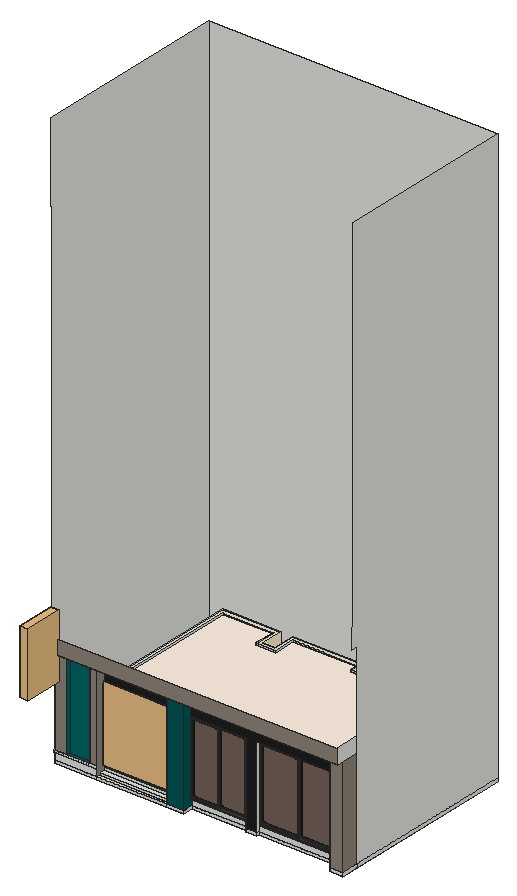
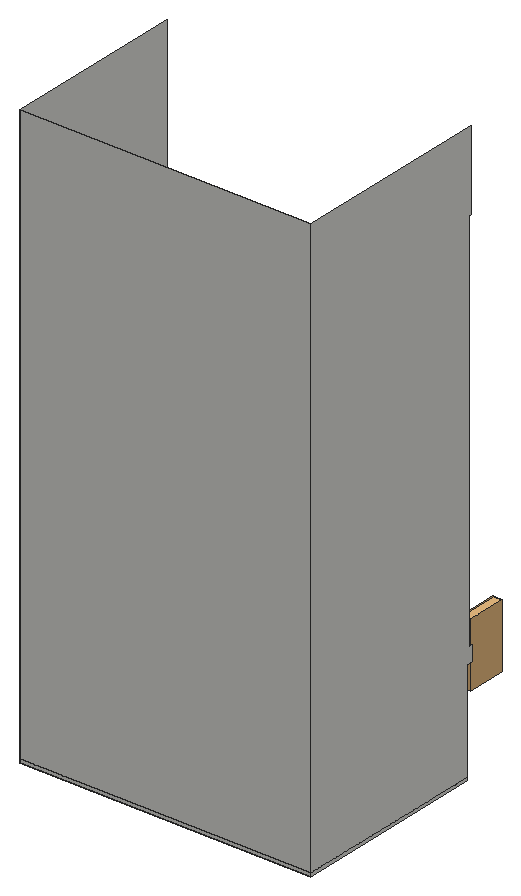
# SketchUp Ruby script. Lengths in inches.
U = 1.inch
M = Sketchup.active_model
def pt(a) = Geom::Point3d.new(a.map { |v| v * U })
def face(e, loops, mat)
  f = e.add_face(loops[0].map { |a| pt(a) })
  loops[1..].each { |l| e.add_face(l.map { |a| pt(a) }).erase! }
  f.material = f.back_material = mat if mat
  f
end
# faces: each face lists its corners as indices into pts; further lists are holes
def faces(e, pts, list, mat = nil) = list.each { |f| face(e, (f[0].is_a?(Array) ? f : [f]).map { |l| l.map { |i| pts[i] } }, mat) }
# xy, xz, yz: faces in a plane at the given z, y or x. An outline is a flat list of corners, or four numbers for a rectangle; further outlines are holes
def ring(l) = l.size == 4 ? [[l[0], l[1]], [l[2], l[1]], [l[2], l[3]], [l[0], l[3]]] : l.each_slice(2).to_a
def flat(e, list, mat, &to3) = list.each { |f| face(e, (f[0].is_a?(Array) ? f : [f]).map { |l| ring(l).map { |u, v| to3.(u, v) } }, mat) }
def xy(e, z, list, mat = nil) = flat(e, list, mat) { |x, y| [x, y, z] }
def xz(e, y, list, mat = nil) = flat(e, list, mat) { |x, z| [x, y, z] }
def yz(e, x, list, mat = nil) = flat(e, list, mat) { |y, z| [x, y, z] }
def lines(e, pts, list) = list.each { |a, b| e.add_line(pt(pts[a]), pt(pts[b])) }
# prism: a flat outline (further loops are holes) pulled along v
def prism(e, loops, v, mat = nil)
  f = face(e, loops, mat); d = Geom::Vector3d.new(v.map { |x| x * U })
  f.pushpull(f.normal.samedirection?(d) ? d.length : -d.length)
end
def box(e, o, s, mat = nil) = prism(e, [[o, [o[0] + s[0], o[1], o[2]], [o[0] + s[0], o[1] + s[1], o[2]], [o[0], o[1] + s[1], o[2]]]], [0, 0, s[2]], mat)
def at(x, y, z, deg = 0) = Geom::Transformation.translation(pt([x, y, z])) * Geom::Transformation.rotation(ORIGIN, Z_AXIS, deg.degrees)
def axes(o, x, y, z) = Geom::Transformation.new([*x, 0, *y, 0, *z, 0, *pt(o).to_a, 1])
def part(name) = M.definitions.add(name)
# library, detail: a bought-in or finely detailed component or shape, given as its bounding box
def library(name, o, s) = part(name).tap { |d| box(d.entities, o, s) }
def detail(e, o, s) = box(e.add_group.entities, o, s)
def put(e, d, t, mat = nil) = e.add_instance(d, t).tap { |i| i.material = mat if mat }
def group(e, t, mat = nil) = e.add_group.tap { |g| g.transformation = t; g.material = mat if mat }.entities
root = M.entities
M.materials.add("Brown Tiles 240cm").color = [174, 145, 135]
M.materials.add("Glass_Tinted_Gray").color = [0, 0, 0]
M.materials["Glass_Tinted_Gray"].alpha = 0.125
M.materials.add("Heather_Band").color = [142, 133, 122]
M.materials.add("[0135_DarkGray]").color = [81, 81, 81]
M.materials.add("[Color C02]").color = [255, 240, 226]
M.materials.add("[Color D01]").color = [255, 242, 204]
M.materials.add("[Color H08]").color = [0, 84, 84]
M.materials.add("[Color H08]1").color = [0, 102, 102]
M.materials.add("[Color M01]1").color = [226, 226, 226]
M.materials.add("[Color M08]").color = [30, 30, 30]
M.materials.add("[Mirror 02]").color = [229, 229, 229]
M.materials.add("[Terrazzo Light Blue]").color = [196, 214, 227]
c1 = part("PENTEK_RP Fineline 50S_Sliding_DoorCase_E1")
box(c1.entities,[0,0,0],[1.51,3.66,99.27],"[0135_DarkGray]")
c2 = part("PENTEK_RP Fineline 50S_SlidingDooe_Case_E2")
box(c2.entities,[0,0,0],[96.25,3.66,1.51],"[0135_DarkGray]")
c3 = part("pentek_RP Fineline 50S_SlidingDoor_Case")
put(c3.entities,c1,at(97.76,0,0))
put(c3.entities,c2,at(1.51,0,0))
put(c3.entities,c1,at(0,0,0))
put(c3.entities,c2,at(1.51,0,97.76))
c4 = part("PENTEK_RP Fineline 50S_SlidingDoor_GlazingBead_2")
box(c4.entities,[0,0,0],[0.56,0.59,94.39],"[0135_DarkGray]")
c5 = part("PENTEK_RP Fineline 50S_SlidingDoor_Glass")
box(c5.entities,[0,0,0],[46.58,0.16,94.39],"Glass_Tinted_Gray")
c6 = part("PENTEK_RP Fineline 50S_SlidingDoor_GlazingBead")
box(c6.entities,[0,0,0],[45.47,0.59,0.56],"[0135_DarkGray]")
c7 = part("PENTEK_RP Fineline 50S_SlidingDoor_Leaf_E1")
xy(c7.entities,0,[[0,0,0.93,1.97],[0.93,1.57,1.49,1.97]],"[0135_DarkGray]")
xy(c7.entities,96.25,[[0,0,0.93,0,0.93,1.57,1.49,1.57,1.49,1.97,0,1.97]],"[0135_DarkGray]")
xz(c7.entities,0,[[0,0,0.93,96.25]],"[0135_DarkGray]")
xz(c7.entities,1.57,[[0.93,0,1.49,95.32],[0.93,95.32,1.49,96.25]],"[0135_DarkGray]")
xz(c7.entities,1.97,[[0,0,1.49,96.25]],"[0135_DarkGray]")
yz(c7.entities,0,[[0,0,1.97,96.25]],"[0135_DarkGray]")
yz(c7.entities,0.93,[[0,0,1.57,0.93],[0,0.93,1.57,95.32],[0,95.32,1.57,96.25]],"[0135_DarkGray]")
yz(c7.entities,1.49,[[1.57,0,1.97,95.32],[1.57,95.32,1.97,96.25]],"[0135_DarkGray]")
c8 = part("PENTEK_RP Fineline 50S_SlidingDoor_Leaf_E2")
xy(c8.entities,0,[[0,0,0,1.57,0.56,1.57,0.56,1.97,46.02,1.97,46.02,1.57,46.58,1.57,46.58,0]],"[0135_DarkGray]")
xy(c8.entities,0.93,[[0,0,46.58,1.57]],"[0135_DarkGray]")
xy(c8.entities,1.49,[[0.56,1.57,46.02,1.97]],"[0135_DarkGray]")
xz(c8.entities,0,[[0,0,46.58,0.93]],"[0135_DarkGray]")
xz(c8.entities,1.57,[[0,0,0.56,0.93],[46.02,0,46.58,0.93],[0.56,0.93,46.02,1.49]],"[0135_DarkGray]")
xz(c8.entities,1.97,[[0.56,0,46.02,1.49]],"[0135_DarkGray]")
yz(c8.entities,0,[[0,0,1.57,0.93]],"[0135_DarkGray]")
yz(c8.entities,0.56,[[1.57,0,1.97,0.93],[1.57,0.93,1.97,1.49]],"[0135_DarkGray]")
yz(c8.entities,46.02,[[1.57,0,1.97,0.93],[1.57,0.93,1.97,1.49]],"[0135_DarkGray]")
yz(c8.entities,46.58,[[0,0,1.57,0.93]],"[0135_DarkGray]")
c9 = part("PENTEK_RP Fineline S_SlidingDoor_Leaf1")
put(c9.entities,c4,at(0.93,0,0.93))
put(c9.entities,c4,at(46.96,0,0.93))
put(c9.entities,c5,at(1.49,1.42,0.93))
put(c9.entities,c6,at(1.49,0,0.93))
put(c9.entities,c5,at(1.49,0.59,0.93),"[Terrazzo Light Blue]")
put(c9.entities,c7,at(0,0,0))
put(c9.entities,c7,axes([48.44,0,0],[-1,0,0],[0,1,0],[0,0,1]))
put(c9.entities,c8,axes([0.93,0,96.25],[1,0,0],[0,1,0],[0,0,-1]))
put(c9.entities,c8,at(0.93,0,0))
put(c9.entities,c6,at(1.49,0,94.77))
c10 = part("PENTEK_RP Fineline 50S_SlidingDoor_Leaf2")
put(c10.entities,c5,at(1.49,1.42,0.93))
put(c10.entities,c6,at(1.49,0,94.77))
put(c10.entities,c4,at(46.96,0,0.93))
put(c10.entities,c5,at(1.49,0.59,0.93),"[Mirror 02]")
put(c10.entities,c4,at(0.93,0,0.93))
put(c10.entities,c7,at(0,0,0))
put(c10.entities,c7,axes([48.44,0,0],[-1,0,0],[0,1,0],[0,0,1]))
put(c10.entities,c6,at(1.49,0,0.93))
put(c10.entities,c8,axes([0.93,0,96.25],[1,0,0],[0,1,0],[0,0,-1]))
put(c10.entities,c8,at(0.93,0,0))
c11 = part("PENTEK - Slimmest Steel Sliding Door / Window\#1")
put(c11.entities,c3,at(0,-1.88,-0.09))
put(c11.entities,c9,at(1.51,-2.27,1.42))
put(c11.entities,c10,at(49.32,-0.3,1.42))
c12 = library("Glass+Door",[0,0,0],[72,3.54,96])
c13 = library("Building Sign 162 041",[-35.6,-7.14,-59.53],[35.45,14.28,119.05])
xy(root,0,[[0,13.61,0,372.45,534.76,372.45,534.76,13.61,510.42,13.61,510.42,32.73,363.26,32.73,363.26,29.02,342.26,29.02,342.26,32.73,239.23,32.73,239.23,13.61]])
xy(root,5.66,[[0,13.61,79,13.61,79,19.17,208.34,19.17,208.34,13.61,239.23,13.61,239.23,32.73,342.26,32.73,342.26,29.02,363.26,29.02,363.26,32.73,510.42,32.73,510.42,13.61,534.76,13.61,534.76,372.45,0,372.45],[79,13.61,208.34,19.17]])
xy(root,9.57,[[79,19.17,208.34,29.02]])
xy(root,14.73,[[79,29.02,208.34,31.95],[239.23,32.73,342.26,34.58],[363.26,32.73,510.42,34.58]])
xy(root,17.05,[[79,29.02,208.34,31.95],[239.23,32.73,342.26,34.58],[363.26,32.73,510.42,34.58]])
xy(root,19.11,[[0,12.67,79,13.61]])
xy(root,19.11,[[79,29.02,208.34,29.02,208.34,37.55,239.23,37.55,239.23,32.73,342.26,32.73,342.26,37.55,363.26,37.55,363.26,32.73,510.42,32.73,510.42,74.25,497.11,74.25,497.11,304.42,361.29,304.42,361.29,287.67,342.26,287.67,342.26,304.42,208.34,304.42,208.34,263.36,186.47,263.36,186.47,304.42,79,304.42]],"Brown Tiles 240cm")
xy(root,23,[[0,12.67,23.3125,13.61],[65.03,12.67,79,13.61]])
xy(root,23,[[23.3125,12.67,65.03,19.67]],"[Color H08]1")
xy(root,152.6,[[85.77,35.79,85.77,297.65,179.69,297.65,179.69,256.58,215.12,256.58,215.12,297.65,335.48,297.65,335.48,280.9,368.07,280.9,368.07,297.65,490.33,297.65,490.33,67.47,503.64,67.47,503.64,35.79,370.03,35.79,370.03,44.32,335.48,44.32,335.48,35.79,246,35.79,246,44.32,201.57,44.32,201.57,35.79]],"[Color C02]")
xy(root,155.66,[[[79,29.02,79,304.42,186.47,304.42,186.47,263.36,208.34,263.36,208.34,304.42,342.26,304.42,342.26,287.67,361.29,287.67,361.29,304.42,497.11,304.42,497.11,74.25,510.42,74.25,510.42,29.02,363.26,29.02,363.26,37.55,342.26,37.55,342.26,29.02,239.23,29.02,239.23,37.55,208.34,37.55,208.34,29.02],[85.77,35.79,201.57,35.79,201.57,44.32,246,44.32,246,35.79,335.48,35.79,335.48,44.32,370.03,44.32,370.03,35.79,503.64,35.79,503.64,67.47,490.33,67.47,490.33,297.65,368.07,297.65,368.07,280.9,335.48,280.9,335.48,297.65,215.12,297.65,215.12,256.58,179.69,256.58,179.69,297.65,85.77,297.65]]])
xy(root,187.02,[[23.3125,13.61,65.03,19.67]],"[Color H08]1")
xy(root,190.91,[[0,1.33,0,13.61,79,13.61,79,29.02,208.34,29.02,208.34,13.61,239.23,13.61,239.23,29.02,510.42,29.02,510.42,13.61,534.76,13.61,534.76,1.33]],"Heather_Band")
xz(root,1.33,[[0,190.91,534.76,216.59]],"Heather_Band")
xz(root,12.67,[[0,19.11,79,23]],"[Color M01]1")
xz(root,13.61,[[79,0,208.34,5.66],[208.34,0,239.23,5.66],[510.42,0,534.76,5.66]])
xz(root,13.61,[[510.42,5.66,534.76,190.91],[0,23,23.3125,23,23.3125,187.02,65.03,187.02,65.03,23,79,23,79,190.91,0,190.91]],"Heather_Band")
xz(root,13.61,[[208.34,5.66,239.23,190.91]],"[Color H08]")
xz(root,13.61,[[0,0,79,5.66],[0,5.66,79,19.11]],"[Color M01]1")
xz(root,19.17,[[79,5.66,208.34,9.57]])
xz(root,19.67,[[23.3125,23,65.03,187.02]],"[Color H08]1")
xz(root,29.02,[[342.26,0,363.26,5.66],[79,9.57,208.34,14.73],[79,17.05,208.34,19.11]])
xz(root,29.02,[[342.26,5.66,363.26,5.66,363.26,155.66,510.42,155.66,510.42,190.91,239.23,190.91,239.23,155.66,342.26,155.66],[79,155.66,208.34,190.91]],"[Color M08]")
xz(root,31.95,[[79,14.73,208.34,17.05]])
xz(root,32.73,[[239.23,0,342.26,5.66],[363.26,0,510.42,5.66],[239.23,5.66,342.26,14.73],[363.26,5.66,510.42,14.73],[239.23,17.05,342.26,19.11],
  [363.26,17.05,510.42,19.11]])
xz(root,34.58,[[239.23,14.73,342.26,17.05],[363.26,14.73,510.42,17.05]])
xz(root,35.79,[[85.77,152.6,201.57,155.66],[246,152.6,335.48,155.66],[370.03,152.6,503.64,155.66]])
xz(root,37.55,[[208.34,19.11,239.23,155.66],[342.26,19.11,363.26,155.66]])
xz(root,44.32,[[201.57,152.6,246,155.66],[335.48,152.6,370.03,155.66]])
xz(root,67.47,[[490.33,152.6,503.64,155.66]])
xz(root,74.25,[[497.11,19.11,510.42,155.66]],"[Color D01]")
xz(root,256.58,[[179.69,152.6,215.12,155.66]])
xz(root,263.36,[[186.47,19.11,208.34,155.66]],"[Color D01]")
xz(root,280.9,[[335.48,152.6,368.07,155.66]])
xz(root,287.67,[[342.26,19.11,361.29,155.66]],"[Color D01]")
xz(root,297.65,[[85.77,152.6,179.69,155.66],[215.12,152.6,335.48,155.66],[368.07,152.6,490.33,155.66]])
xz(root,304.42,[[79,19.11,186.47,155.66],[208.34,19.11,342.26,155.66],[361.29,19.11,497.11,155.66]],"[Color D01]")
xz(root,372.45,[[0,0,534.76,5.66],[0,5.66,534.76,1076]])
yz(root,0,[[13.61,0,372.45,5.66],[13.61,5.66,13.61,19.11,12.67,19.11,12.67,23,13.61,23,13.61,190.91,1.33,190.91,1.33,219.25,8.08,219.25,8.08,929.63,4.77,929.63,4.77,1076,372.45,1076,372.45,5.66]])
yz(root,23.3125,[[13.61,23,19.67,187.02]],"[Color H08]1")
yz(root,65.03,[[13.61,23,19.67,187.02]],"[Color H08]1")
yz(root,79,[[29.02,14.73,31.95,17.05]])
yz(root,79,[[13.61,5.66,19.17,5.66,19.17,9.57,29.02,9.57,29.02,190.91,13.61,190.91,13.61,23,12.67,23,12.67,19.11,13.61,19.11]],"Heather_Band")
yz(root,79,[[29.02,19.11,304.42,155.66]],"[Color D01]")
yz(root,85.77,[[35.79,152.6,297.65,155.66]])
yz(root,179.69,[[256.58,152.6,297.65,155.66]])
yz(root,186.47,[[263.36,19.11,304.42,155.66]],"[Color D01]")
yz(root,201.57,[[35.79,152.6,44.32,155.66]])
yz(root,208.34,[[263.36,19.11,304.42,155.66]],"[Color D01]")
yz(root,208.34,[[13.61,5.66,13.61,190.91,29.02,190.91,29.02,155.66,37.55,155.66,37.55,19.11,29.02,19.11,29.02,17.05,31.95,17.05,31.95,14.73,29.02,14.73,29.02,9.57,19.17,9.57,19.17,5.66]],"[Color H08]")
yz(root,215.12,[[256.58,152.6,297.65,155.66]])
yz(root,239.23,[[13.61,0,32.73,5.66]])
yz(root,239.23,[[13.61,5.66,32.73,5.66,32.73,14.73,34.58,14.73,34.58,17.05,32.73,17.05,32.73,19.11,37.55,19.11,37.55,155.66,29.02,155.66,29.02,190.91,13.61,190.91]],"[Color H08]")
yz(root,246,[[35.79,152.6,44.32,155.66]])
yz(root,335.48,[[35.79,152.6,44.32,155.66],[280.9,152.6,297.65,155.66]])
yz(root,342.26,[[29.02,0,32.73,5.66],[29.02,5.66,29.02,155.66,37.55,155.66,37.55,19.11,32.73,19.11,32.73,17.05,34.58,17.05,34.58,14.73,32.73,14.73,32.73,5.66]])
yz(root,342.26,[[287.67,19.11,304.42,155.66]],"[Color D01]")
yz(root,361.29,[[287.67,19.11,304.42,155.66]])
yz(root,363.26,[[29.02,0,32.73,5.66],[29.02,5.66,32.73,5.66,32.73,14.73,34.58,14.73,34.58,17.05,32.73,17.05,32.73,19.11,37.55,19.11,37.55,155.66,29.02,155.66]])
yz(root,368.07,[[280.9,152.6,297.65,155.66]])
yz(root,370.03,[[35.79,152.6,44.32,155.66]])
yz(root,490.33,[[67.47,152.6,297.65,155.66]])
yz(root,497.11,[[74.25,19.11,304.42,155.66]],"[Color D01]")
yz(root,503.64,[[35.79,152.6,67.47,155.66]])
yz(root,510.42,[[13.61,0,29.02,5.66],[29.02,0,32.73,5.66],[13.61,5.66,29.02,190.91],[29.02,5.66,29.02,155.66,74.25,155.66,74.25,19.11,32.73,19.11,32.73,17.05,34.58,17.05,34.58,14.73,32.73,14.73,32.73,5.66]])
yz(root,534.76,[[13.61,0,46.67,5.66],[46.67,0,372.45,5.66],[46.67,5.66,372.45,5.66,372.45,1076,35.95,1076,35.95,403.08,34.05,403.08,34.05,366.625,46.67,366.625],[1.33,190.91,46.67,219.25]])
yz(root,534.76,[[13.61,5.66,46.67,190.91]],"Heather_Band")
put(root,c11,axes([239.23,31.84,19.1875],[1.04,0,0],[0,1,0],[0,0,1.37602]))
put(root,c11,axes([365.06,34.61,19.23],[1.4664,0,0],[0,1,0],[0,0,1.37602]))
put(root,c12,axes([79.01,27.29,19.11],[1.7973,0,0],[0,1.45,0],[0,0,1.45]))
put(root,c13,axes([7.5,5.07,204.24],[0,2.01,0],[-1.05,0,0],[0,0,1]))
